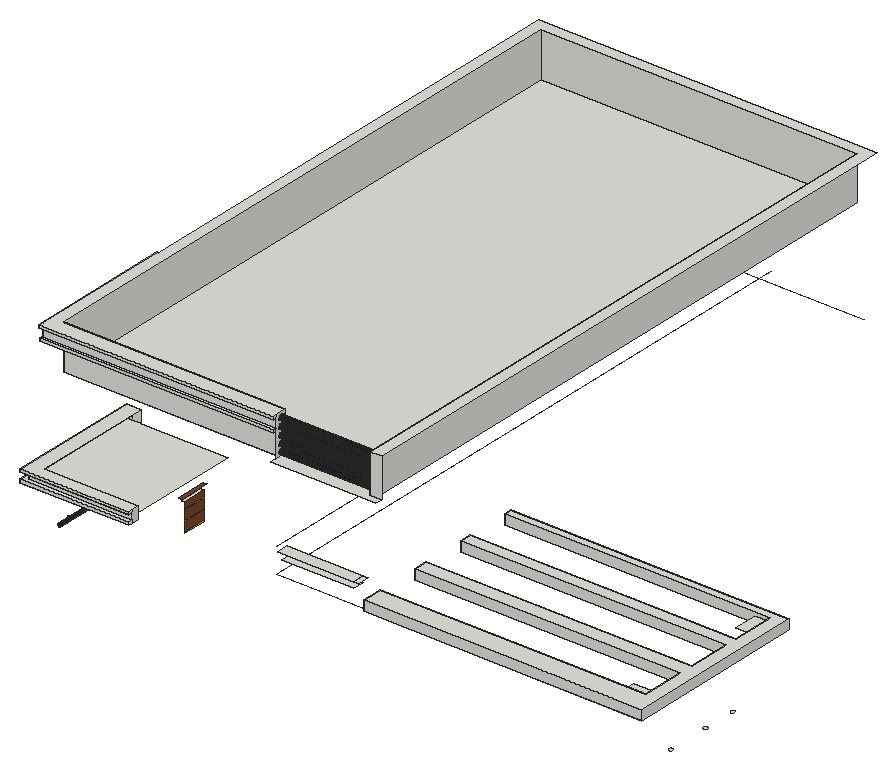
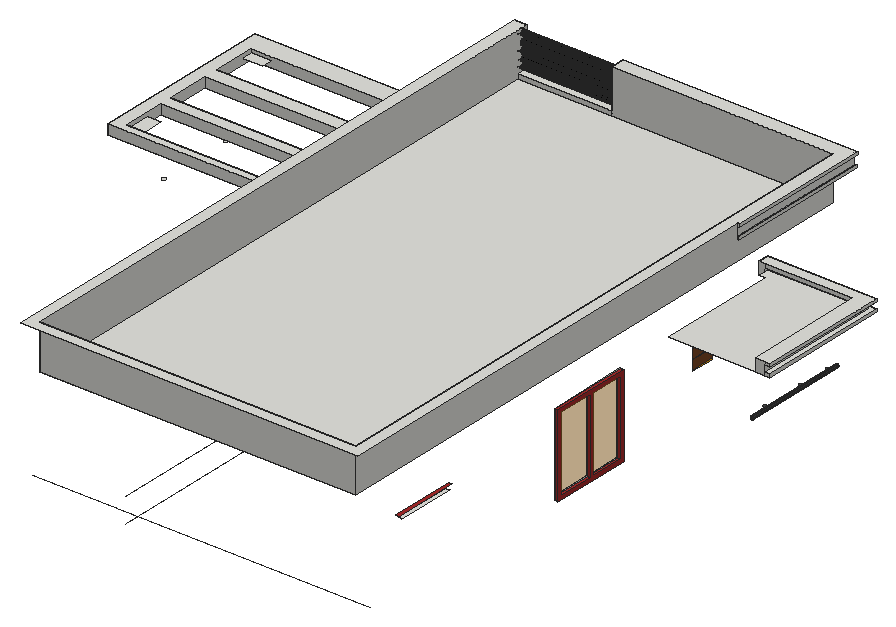
# SketchUp Ruby script. Lengths in inches.
U = 1.inch
M = Sketchup.active_model
def pt(a) = Geom::Point3d.new(a.map { |v| v * U })
def face(e, loops, mat)
  f = e.add_face(loops[0].map { |a| pt(a) })
  loops[1..].each { |l| e.add_face(l.map { |a| pt(a) }).erase! }
  f.material = f.back_material = mat if mat
  f
end
# faces: each face lists its corners as indices into pts; further lists are holes
def faces(e, pts, list, mat = nil) = list.each { |f| face(e, (f[0].is_a?(Array) ? f : [f]).map { |l| l.map { |i| pts[i] } }, mat) }
# xy, xz, yz: faces in a plane at the given z, y or x. An outline is a flat list of corners, or four numbers for a rectangle; further outlines are holes
def ring(l) = l.size == 4 ? [[l[0], l[1]], [l[2], l[1]], [l[2], l[3]], [l[0], l[3]]] : l.each_slice(2).to_a
def flat(e, list, mat, &to3) = list.each { |f| face(e, (f[0].is_a?(Array) ? f : [f]).map { |l| ring(l).map { |u, v| to3.(u, v) } }, mat) }
def xy(e, z, list, mat = nil) = flat(e, list, mat) { |x, y| [x, y, z] }
def xz(e, y, list, mat = nil) = flat(e, list, mat) { |x, z| [x, y, z] }
def yz(e, x, list, mat = nil) = flat(e, list, mat) { |y, z| [x, y, z] }
def lines(e, pts, list) = list.each { |a, b| e.add_line(pt(pts[a]), pt(pts[b])) }
# prism: a flat outline (further loops are holes) pulled along v
def prism(e, loops, v, mat = nil)
  f = face(e, loops, mat); d = Geom::Vector3d.new(v.map { |x| x * U })
  f.pushpull(f.normal.samedirection?(d) ? d.length : -d.length)
end
def box(e, o, s, mat = nil) = prism(e, [[o, [o[0] + s[0], o[1], o[2]], [o[0] + s[0], o[1] + s[1], o[2]], [o[0], o[1] + s[1], o[2]]]], [0, 0, s[2]], mat)
def at(x, y, z, deg = 0) = Geom::Transformation.translation(pt([x, y, z])) * Geom::Transformation.rotation(ORIGIN, Z_AXIS, deg.degrees)
def axes(o, x, y, z) = Geom::Transformation.new([*x, 0, *y, 0, *z, 0, *pt(o).to_a, 1])
def part(name) = M.definitions.add(name)
# library, detail: a bought-in or finely detailed component or shape, given as its bounding box
def library(name, o, s) = part(name).tap { |d| box(d.entities, o, s) }
def detail(e, o, s) = box(e.add_group.entities, o, s)
def put(e, d, t, mat = nil) = e.add_instance(d, t).tap { |i| i.material = mat if mat }
def group(e, t, mat = nil) = e.add_group.tap { |g| g.transformation = t; g.material = mat if mat }.entities
root = M.entities
M.materials.add("[0018_Brown]").color = [165, 42, 42]
M.materials.add("[0038_Orange]").color = [255, 165, 0]
M.materials.add("[0137_Black]").color = [71, 71, 71]
M.materials.add("[0137_Black]1").color = [0, 0, 0]
M.materials.add("[Translucent Glass Gray]").color = [191, 123, 24]
M.materials["[Translucent Glass Gray]"].alpha = 0.5
M.materials.add("[Wood Veneer 01]").color = [120, 70, 37]
prism(root,[[[512.421,0,493.967],[286.171,0,493.967],[286.171,12.1875,493.967],[286.171,16.939,493.967],[501.796,16.939,493.967],[501.796,51.752,493.967],[286.171,51.752,493.967],[286.171,63.752,493.967],[501.796,63.752,493.967],[501.796,98.564,493.967],[286.171,98.564,493.967],[286.171,108.439,493.967],[501.796,108.439,493.967],[501.796,143.252,493.967],[286.171,143.252,493.967],[286.171,149.476,493.967],[512.421,149.476,493.967]]],[0,0,8])
xy(root,448.181,[[499.408,44.29,499.78,44.339,500.127,44.482,500.424,44.711,500.653,45.008,500.796,45.355,500.845,45.727,500.796,46.099,500.653,46.446,500.424,46.744,500.127,46.972,499.78,47.116,499.408,47.165,499.036,47.116,498.689,46.972,498.391,46.744,498.163,46.446,498.019,46.099,497.97,45.727,498.019,45.355,498.163,45.008,498.391,44.711,498.689,44.482,499.036,44.339],[499.408,79.415,499.78,79.464,500.127,79.607,500.424,79.836,500.653,80.133,500.796,80.48,500.845,80.852,500.796,81.224,500.653,81.571,500.424,81.869,500.127,82.097,499.78,82.241,499.408,82.29,499.036,82.241,498.689,82.097,498.391,81.869,498.163,81.571,498.019,81.224,497.97,80.852,498.019,80.48,498.163,80.133,498.391,79.836,498.689,79.607,499.036,79.464],[499.408,107.04,499.78,107.089,500.127,107.232,500.424,107.461,500.653,107.758,500.796,108.105,500.845,108.477,500.796,108.849,500.653,109.196,500.424,109.494,500.127,109.722,499.78,109.866,499.408,109.915,499.036,109.866,498.689,109.722,498.391,109.494,498.163,109.196,498.019,108.849,497.97,108.477,498.019,108.105,498.163,107.758,498.391,107.461,498.689,107.232,499.036,107.089]])
xy(root,450.401,[[15.224,38.964,15.465,38.996,15.69,39.089,15.882,39.237,16.03,39.429,16.123,39.654,16.155,39.895,16.123,40.135,16.03,40.36,15.882,40.552,15.69,40.7,15.465,40.793,15.224,40.825,14.984,40.793,14.759,40.7,14.566,40.552,14.419,40.36,14.326,40.135,14.294,39.895,14.326,39.654,14.419,39.429,14.566,39.237,14.759,39.089,14.984,38.996],[15.849,65.839,16.09,65.871,16.315,65.964,16.507,66.112,16.655,66.304,16.748,66.529,16.78,66.77,16.748,67.01,16.655,67.235,16.507,67.427,16.315,67.575,16.09,67.668,15.849,67.7,15.609,67.668,15.384,67.575,15.191,67.427,15.044,67.235,14.951,67.01,14.919,66.77,14.951,66.529,15.044,66.304,15.191,66.112,15.384,65.964,15.609,65.871],[15.849,101.902,16.09,101.933,16.315,102.026,16.507,102.174,16.655,102.367,16.748,102.591,16.78,102.832,16.748,103.073,16.655,103.297,16.507,103.49,16.315,103.638,16.09,103.731,15.849,103.762,15.609,103.731,15.384,103.638,15.191,103.49,15.044,103.297,14.951,103.073,14.919,102.832,14.951,102.591,15.044,102.367,15.191,102.174,15.384,102.026,15.609,101.933]],"[0137_Black]")
xy(root,470.089,[[79.845,73.086,82.845,92.211]])
xy(root,473.089,[[79.845,70.086,82.845,95.211]],"[Wood Veneer 01]")
xy(root,479.029,[[8.875,254.471,11.875,321.346]],"[0018_Brown]")
xy(root,482.029,[[8.875,257.471,11.875,285.627],[8.875,287.909,11.875,318.346]],"[0018_Brown]")
xy(root,483,[[[0,9.1875,0,117.1875,11.875,117.1875,11.875,116.75,82.845,116.75,82.845,18.1875,88.408,18.1875,88.408,9.1875],[11.9375,19,16.875,30.25]],[11.9375,19,16.875,30.25],[284.046,22.046,284.046,22.066,284.415,22.0625,285.29,22.0625,285.29,22.054,286.171,22.046],[284.046,22.046,284.415,22.054],[284.415,22.046,285.29,22.054],
  [285.29,22.046,286.171,22.046,285.29,22.054],[284.046,22.054,284.415,22.0625],[284.415,22.054,285.29,22.054,284.415,22.0625],[285.29,22.054,285.29,22.0625,284.415,22.0625],[284.046,22.0625,284.415,22.0625,284.046,22.066]])
xy(root,485.689,[[0,9.1875,88.408,9.1875,88.408,12.1875,4.125,12.1875,4.125,117.1875,0,117.1875]])
xy(root,490.904,[[0,9.1875,0,117.1875,4.125,117.1875,4.125,12.1875,88.408,12.1875,88.408,9.1875]])
xy(root,493.0625,[[0,9.1875,88.408,9.1875,88.408,18.1875,11.875,18.1875,11.875,117.1875,0,117.1875]])
xy(root,499.431,[[484.5625,1.0625,510.6875,26.4375],[490.125,122.75,510.6875,143.77]])
xy(root,505.684,[[217.107,3.1875,275.758,12.1875]])
xy(root,510.503,[[213.982,3.1875,275.758,12.1875]])
xy(root,510.53,[[275.758,3.1875,279.919,12.1875]])
xy(root,536.147,[[8.875,431.778,11.875,479.716]])
xy(root,539.147,[[8.875,428.778,11.875,482.716]],"[0018_Brown]")
xy(root,542.904,[[8.875,257.471,11.875,285.627],[8.875,287.909,11.875,318.346]],"[0018_Brown]")
xy(root,545.904,[[8.875,254.471,11.875,321.346]],"[0018_Brown]")
xy(root,563.125,[[20.875,27.1875,277.171,511.875]])
xy(root,567.219,[[200.791,12.1875,286.171,12.1875,286.171,18.1875,277.171,18.1875,277.171,27.1875,200.791,27.1875]])
xy(root,587.3125,[[10.75,15.1875,10.75,135.0625,11.875,135.0625,11.875,18.1875,200.791,18.1875,200.791,15.1875]])
xy(root,589.538,[[10.75,15.1875,200.791,15.1875,200.791,17.5625,11.875,17.5625,11.875,135.0625,10.75,135.0625],[11.875,17.5625,200.791,18.1875]])
xy(root,596.571,[[10.25,15.1875,10.25,135.0625,11.875,135.0625,11.875,17.5625,200.791,17.5625,200.791,15.1875]])
xy(root,599.125,[[10.25,15.1875,200.791,15.1875,200.791,27.1875,20.875,27.1875,20.875,511.875,277.171,511.875,277.171,18.1875,286.171,18.1875,286.171,520.875,11.875,520.875,11.875,135.0625,10.25,135.0625]])
xz(root,9.1875,[[0,483,88.408,485.689],[0,490.904,88.408,493.0625]])
xz(root,12.1875,[[4.125,485.689,88.408,490.904]])
xz(root,15.1875,[[10.75,587.3125,200.791,589.538],[10.25,596.571,200.791,599.125]])
xz(root,17.5625,[[11.875,589.538,200.791,596.571]])
xz(root,18.1875,[[277.171,567.219,286.171,599.125],[11.875,587.243,200.791,587.3125],[11.875,587.3125,200.791,589.538]])
xz(root,27.1875,[[20.875,563.125,200.791,599.125],[200.791,563.125,277.171,567.219]])
xz(root,117.1875,[[0,483,4.125,485.689],[4.125,483,11.875,493.0625],[0,490.904,4.125,493.0625]])
xz(root,135.0625,[[10.75,587.3125,11.875,589.538],[10.25,596.571,11.875,599.125]])
xz(root,254.471,[[8.875,479.029,11.875,545.904]],"[0018_Brown]")
xz(root,257.471,[[8.875,482.029,11.875,542.904]],"[0018_Brown]")
xz(root,285.627,[[8.875,482.029,11.875,542.904]],"[0018_Brown]")
xz(root,287.909,[[8.875,482.029,11.875,542.904]],"[0018_Brown]")
xz(root,318.346,[[8.875,482.029,11.875,542.904]],"[0018_Brown]")
xz(root,321.346,[[8.875,479.029,11.875,545.904]],"[0018_Brown]")
xz(root,511.875,[[20.875,563.125,277.171,599.125]])
yz(root,0,[[9.1875,483,117.1875,485.689],[9.1875,490.904,117.1875,493.0625]])
yz(root,4.125,[[12.1875,485.689,117.1875,490.904]])
yz(root,8.875,[[[254.471,479.029,321.346,545.904],[287.909,482.029,318.346,542.904],[257.471,482.029,285.627,542.904]]],"[0018_Brown]")
yz(root,10.25,[[15.1875,596.571,135.0625,599.125]])
yz(root,10.75,[[15.1875,587.3125,135.0625,589.538]])
yz(root,11.875,[[[254.471,479.029,321.346,545.904],[287.909,482.029,318.346,542.904],[257.471,482.029,285.627,542.904]],[18.1875,587.3125,135.0625,589.538],[17.5625,589.538,135.0625,596.571]])
yz(root,11.875,[[257.471,482.029,285.627,542.904],[287.909,482.029,318.346,542.904]],"[Translucent Glass Gray]")
yz(root,20.875,[[27.1875,563.125,511.875,599.125]])
yz(root,82.845,[[73.086,447.376,92.211,448.489],[73.086,455.688,92.211,456.802],[73.086,464.001,92.211,465.114]],"[0038_Orange]")
yz(root,82.845,[[73.086,448.489,92.211,455.688],[73.086,456.802,92.211,464.001],[73.086,465.114,92.211,470.089]],"[Wood Veneer 01]")
yz(root,88.408,[[9.1875,483,12.1875,485.689],[12.1875,483,18.1875,493.0625],[9.1875,490.904,12.1875,493.0625]])
yz(root,200.791,[[[18.1875,567.219,27.1875,567.219,27.1875,599.125,18.1875,599.125,18.1875,596.571,17.5625,596.571,17.5625,589.538,18.1875,589.538],[22.313,593.302,21.763,593.374,21.251,593.586,20.811,593.924,20.473,594.364,20.261,594.877,20.188,595.427,20.261,595.977,20.473,596.489,20.811,596.929,21.251,597.267,21.763,597.479,22.313,597.552,22.863,597.479,23.376,597.267,23.816,596.929,24.154,596.489,24.366,595.977,24.438,595.427,24.366,594.877,24.154,594.364,23.816,593.924,23.376,593.586,22.863,593.374],[22.313,587.052,21.763,587.124,21.251,587.336,20.811,587.674,20.473,588.114,20.261,588.627,20.188,589.177,20.261,589.727,20.473,590.239,20.811,590.679,21.251,591.017,21.763,591.229,22.313,591.302,22.863,591.229,23.376,591.017,23.816,590.679,24.154,590.239,24.366,589.727,24.438,589.177,24.366,588.627,24.154,588.114,23.816,587.674,23.376,587.336,22.863,587.124],[22.313,580.802,21.763,580.874,21.251,581.086,20.811,581.424,20.473,581.864,20.261,582.377,20.188,582.927,20.261,583.477,20.473,583.989,20.811,584.429,21.251,584.767,21.763,584.979,22.313,585.052,22.863,584.979,23.376,584.767,23.816,584.429,24.154,583.989,24.366,583.477,24.438,582.927,24.366,582.377,24.154,581.864,23.816,581.424,23.376,581.086,22.863,580.874],[22.313,574.552,21.763,574.624,21.251,574.836,20.811,575.174,20.473,575.614,20.261,576.127,20.188,576.677,20.261,577.227,20.473,577.739,20.811,578.179,21.251,578.517,21.763,578.729,22.313,578.802,22.863,578.729,23.376,578.517,23.816,578.179,24.154,577.739,24.366,577.227,24.438,576.677,24.366,576.127,24.154,575.614,23.816,575.174,23.376,574.836,22.863,574.624]],[15.1875,587.3125,18.1875,589.538],[15.1875,596.571,18.1875,599.125]])
yz(root,275.758,[[3.1875,510.503,12.1875,510.53]])
yz(root,277.171,[[[27.1875,563.125,27.1875,567.219,18.1875,567.219,18.1875,599.125,511.875,599.125,511.875,563.125],[22.313,587.052,22.863,587.124,23.376,587.336,23.816,587.674,24.154,588.114,24.366,588.627,24.438,589.177,24.366,589.727,24.154,590.239,23.816,590.679,23.376,591.017,22.863,591.229,22.313,591.302,21.763,591.229,21.251,591.017,20.811,590.679,20.473,590.239,20.261,589.727,20.188,589.177,20.261,588.627,20.473,588.114,20.811,587.674,21.251,587.336,21.763,587.124]]])
yz(root,279.354,[[22.313,574.552,22.863,574.624,23.376,574.836,23.816,575.174,24.154,575.614,24.366,576.127,24.438,576.677,24.366,577.227,24.154,577.739,23.816,578.179,23.376,578.517,22.863,578.729,22.313,578.802,21.763,578.729,21.251,578.517,20.811,578.179,20.473,577.739,20.261,577.227,20.188,576.677,20.261,576.127,20.473,575.614,20.811,575.174,21.251,574.836,21.763,574.624],[22.313,580.802,22.863,580.874,23.376,581.086,23.816,581.424,24.154,581.864,24.366,582.377,24.438,582.927,24.366,583.477,24.154,583.989,23.816,584.429,23.376,584.767,22.863,584.979,22.313,585.052,21.763,584.979,21.251,584.767,20.811,584.429,20.473,583.989,20.261,583.477,20.188,582.927,20.261,582.377,20.473,581.864,20.811,581.424,21.251,581.086,21.763,580.874]])
yz(root,279.416,[[22.313,593.302,22.863,593.374,23.376,593.586,23.816,593.924,24.154,594.364,24.366,594.877,24.438,595.427,24.366,595.977,24.154,596.489,23.816,596.929,23.376,597.267,22.863,597.479,22.313,597.552,21.763,597.479,21.251,597.267,20.811,596.929,20.473,596.489,20.261,595.977,20.188,595.427,20.261,594.877,20.473,594.364,20.811,593.924,21.251,593.586,21.763,593.374]])
p = [[14.598,30.25,447.006],[14.311,30.25,447.125],[14.311,116.75,447.125],[14.598,116.75,447.006],[14.905,30.25,446.966],[14.905,116.75,446.966],
  [15.212,30.25,447.006],[15.212,116.75,447.006],[15.499,30.25,447.125],[15.499,116.75,447.125],[14.065,30.25,447.314],[14.065,116.75,447.314],
  [15.745,30.25,447.314],[15.745,116.75,447.314],[13.876,30.25,447.56],[13.876,116.75,447.56],[15.933,30.25,447.56],[15.933,116.75,447.56],
  [13.758,30.25,447.846],[13.758,116.75,447.846],[16.052,30.25,447.846],[16.052,116.75,447.846],[13.717,30.25,448.153],[13.717,116.75,448.153],
  [16.092,30.25,448.153],[16.092,116.75,448.153],[13.758,30.25,448.461],[13.758,116.75,448.461],[16.052,30.25,448.461],[16.052,116.75,448.461],
  [13.876,30.25,448.747],[13.876,116.75,448.747],[15.933,30.25,448.747],[15.933,116.75,448.747],[14.065,30.25,448.993],[14.065,116.75,448.993],
  [15.745,30.25,448.993],[15.745,116.75,448.993],[14.311,30.25,449.182],[14.311,116.75,449.182],[15.499,30.25,449.182],[15.499,116.75,449.182],
  [14.598,30.25,449.3],[14.598,116.75,449.3],[15.212,30.25,449.3],[15.212,116.75,449.3],[14.905,30.25,449.341],[14.905,116.75,449.341],
  [200.791,21.763,569.062],[200.791,22.313,568.989],[279.354,22.313,568.989],[279.354,21.763,569.062],[200.791,22.863,569.062],[279.354,22.863,569.062],
  [200.791,21.251,569.274],[279.354,21.251,569.274],[200.791,23.376,569.274],[279.354,23.376,569.274],[200.791,20.811,569.612],[279.354,20.811,569.612],
  [200.791,23.816,569.612],[279.354,23.816,569.612],[200.791,20.473,570.052],[279.354,20.473,570.052],[200.791,24.154,570.052],[279.354,24.154,570.052],
  [200.791,20.261,570.564],[279.354,20.261,570.564],[200.791,24.366,570.564],[279.354,24.366,570.564],[200.791,20.188,571.114],[279.354,20.188,571.114],
  [200.791,24.438,571.114],[279.354,24.438,571.114],[200.791,20.261,571.664],[279.354,20.261,571.664],[200.791,24.366,571.664],[279.354,24.366,571.664],
  [200.791,20.473,572.177],[279.354,20.473,572.177],[200.791,24.154,572.177],[279.354,24.154,572.177],[200.791,20.811,572.617],[279.354,20.811,572.617],
  [200.791,23.816,572.617],[279.354,23.816,572.617],[200.791,21.251,572.954],[279.354,21.251,572.954],[200.791,23.376,572.954],[279.354,23.376,572.954],
  [200.791,21.763,573.167],[279.354,21.763,573.167],[200.791,22.863,573.167],[279.354,22.863,573.167],[200.791,22.313,573.239],[279.354,22.313,573.239],
  [200.791,21.251,574.836],[200.791,21.763,574.624],[279.354,21.763,574.624],[279.354,21.251,574.836],[200.791,22.313,574.552],[279.354,22.313,574.552],
  [200.791,22.863,574.624],[279.354,22.863,574.624],[200.791,23.376,574.836],[279.354,23.376,574.836],[200.791,20.811,575.174],[279.354,20.811,575.174],
  [200.791,23.816,575.174],[279.354,23.816,575.174],[200.791,20.473,575.614],[279.354,20.473,575.614],[200.791,24.154,575.614],[279.354,24.154,575.614],
  [200.791,20.261,576.127],[279.354,20.261,576.127],[200.791,24.366,576.127],[279.354,24.366,576.127],[200.791,20.188,576.677],[279.354,20.188,576.677],
  [200.791,24.438,576.677],[279.354,24.438,576.677],[200.791,20.261,577.227],[279.354,20.261,577.227],[200.791,24.366,577.227],[279.354,24.366,577.227],
  [200.791,20.473,577.739],[279.354,20.473,577.739],[200.791,24.154,577.739],[279.354,24.154,577.739],[200.791,20.811,578.179],[279.354,20.811,578.179],
  [200.791,23.816,578.179],[279.354,23.816,578.179],[200.791,21.251,578.517],[279.354,21.251,578.517],[200.791,23.376,578.517],[279.354,23.376,578.517],
  [200.791,21.763,578.729],[279.354,21.763,578.729],[200.791,22.863,578.729],[279.354,22.863,578.729],[200.791,22.313,578.802],[279.354,22.313,578.802],
  [200.791,21.763,580.874],[200.791,22.313,580.802],[279.354,22.313,580.802],[279.354,21.763,580.874],[200.791,22.863,580.874],[279.354,22.863,580.874],
  [200.791,21.251,581.086],[279.354,21.251,581.086],[200.791,23.376,581.086],[279.354,23.376,581.086],[200.791,20.811,581.424],[279.354,20.811,581.424],
  [200.791,23.816,581.424],[279.354,23.816,581.424],[200.791,20.473,581.864],[279.354,20.473,581.864],[200.791,24.154,581.864],[279.354,24.154,581.864],
  [200.791,20.261,582.377],[279.354,20.261,582.377],[200.791,24.366,582.377],[279.354,24.366,582.377],[200.791,20.188,582.927],[279.354,20.188,582.927],
  [200.791,24.438,582.927],[279.354,24.438,582.927],[200.791,20.261,583.477],[279.354,20.261,583.477],[200.791,24.366,583.477],[279.354,24.366,583.477],
  [200.791,20.473,583.989],[279.354,20.473,583.989],[200.791,24.154,583.989],[279.354,24.154,583.989],[200.791,20.811,584.429],[279.354,20.811,584.429],
  [200.791,23.816,584.429],[279.354,23.816,584.429],[200.791,21.251,584.767],[279.354,21.251,584.767],[200.791,23.376,584.767],[279.354,23.376,584.767],
  [200.791,21.763,584.979],[279.354,21.763,584.979],[200.791,22.863,584.979],[279.354,22.863,584.979],[200.791,22.313,585.052],[279.354,22.313,585.052],
  [200.791,21.251,587.336],[200.791,21.763,587.124],[277.171,21.763,587.124],[277.171,21.251,587.336],[200.791,22.313,587.052],[277.171,22.313,587.052],
  [200.791,22.863,587.124],[277.171,22.863,587.124],[200.791,23.376,587.336],[277.171,23.376,587.336],[200.791,20.811,587.674],[277.171,20.811,587.674],
  [200.791,23.816,587.674],[277.171,23.816,587.674],[200.791,20.473,588.114],[277.171,20.473,588.114],[200.791,24.154,588.114],[277.171,24.154,588.114],
  [200.791,20.261,588.627],[277.171,20.261,588.627],[200.791,24.366,588.627],[277.171,24.366,588.627],[200.791,20.188,589.177],[277.171,20.188,589.177],
  [200.791,24.438,589.177],[277.171,24.438,589.177],[200.791,20.261,589.727],[277.171,20.261,589.727],[200.791,24.366,589.727],[277.171,24.366,589.727],
  [200.791,20.473,590.239],[277.171,20.473,590.239],[200.791,24.154,590.239],[277.171,24.154,590.239],[200.791,20.811,590.679],[277.171,20.811,590.679],
  [200.791,23.816,590.679],[277.171,23.816,590.679],[200.791,21.251,591.017],[277.171,21.251,591.017],[200.791,23.376,591.017],[277.171,23.376,591.017],
  [200.791,21.763,591.229],[277.171,21.763,591.229],[200.791,22.863,591.229],[277.171,22.863,591.229],[200.791,22.313,591.302],[277.171,22.313,591.302],
  [200.791,21.763,593.374],[200.791,22.313,593.302],[279.416,22.313,593.302],[279.416,21.763,593.374],[200.791,22.863,593.374],[279.416,22.863,593.374],
  [200.791,21.251,593.586],[279.416,21.251,593.586],[200.791,23.376,593.586],[279.416,23.376,593.586],[200.791,20.811,593.924],[279.416,20.811,593.924],
  [200.791,23.816,593.924],[279.416,23.816,593.924],[200.791,20.473,594.364],[279.416,20.473,594.364],[200.791,24.154,594.364],[279.416,24.154,594.364],
  [200.791,20.261,594.877],[279.416,20.261,594.877],[200.791,24.366,594.877],[279.416,24.366,594.877],[200.791,20.188,595.427],[279.416,20.188,595.427],
  [200.791,24.438,595.427],[279.416,24.438,595.427],[200.791,20.261,595.977],[279.416,20.261,595.977],[200.791,24.366,595.977],[279.416,24.366,595.977],
  [200.791,20.473,596.489],[279.416,20.473,596.489],[200.791,24.154,596.489],[279.416,24.154,596.489],[200.791,20.811,596.929],[279.416,20.811,596.929],
  [200.791,23.816,596.929],[279.416,23.816,596.929],[200.791,21.251,597.267],[279.416,21.251,597.267],[200.791,23.376,597.267],[279.416,23.376,597.267],
  [200.791,21.763,597.479],[279.416,21.763,597.479],[200.791,22.863,597.479],[279.416,22.863,597.479],[200.791,22.313,597.552],[279.416,22.313,597.552],
  [200.791,18.1875,483],[286.171,18.1875,483],[200.791,508.3125,483],[200.791,18.1875,503.125],[200.791,520.875,503.125],[11.875,30.25,483],
  [11.9375,30.25,483],[4.125,12.1875,483],[4.125,12.1875,485.689],[275.758,12.1875,505.684],[275.758,12.1875,510.503],[11.875,508.3125,483],
  [286.171,508.3125,483],[200.791,520.875,483],[11.875,18.1875,596.571],[11.875,18.1875,599.125]]
faces(root,p,[[0,1,2,3],[4,0,3,5],[6,4,5,7],[8,6,7,9],[1,10,11,2],[12,8,9,13],[10,14,15,11],[16,12,13,17],
  [14,18,19,15],[20,16,17,21],[18,22,23,19],[24,20,21,25],[22,26,27,23],[28,24,25,29],[26,30,31,27],[32,28,29,33],
  [30,34,35,31],[36,32,33,37],[34,38,39,35],[40,36,37,41],[38,42,43,39],[44,40,41,45],[42,46,47,43],[46,44,45,47]],"[0137_Black]")
faces(root,p,[[48,49,50,51],[49,52,53,50],[54,48,51,55],[52,56,57,53],[58,54,55,59],[56,60,61,57],[62,58,59,63],[60,64,65,61],
  [66,62,63,67],[64,68,69,65],[70,66,67,71],[68,72,73,69],[74,70,71,75],[72,76,77,73],[78,74,75,79],[76,80,81,77],
  [82,78,79,83],[80,84,85,81],[86,82,83,87],[84,88,89,85],[90,86,87,91],[88,92,93,89],[94,90,91,95],[92,94,95,93],
  [96,97,98,99],[97,100,101,98],[100,102,103,101],[102,104,105,103],[106,96,99,107],[104,108,109,105],[110,106,107,111],[108,112,113,109],
  [114,110,111,115],[112,116,117,113],[118,114,115,119],[116,120,121,117],[122,118,119,123],[120,124,125,121],[126,122,123,127],[124,128,129,125],
  [130,126,127,131],[128,132,133,129],[134,130,131,135],[132,136,137,133],[138,134,135,139],[136,140,141,137],[142,138,139,143],[140,142,143,141],
  [144,145,146,147],[145,148,149,146],[150,144,147,151],[148,152,153,149],[154,150,151,155],[152,156,157,153],[158,154,155,159],[156,160,161,157],
  [162,158,159,163],[160,164,165,161],[166,162,163,167],[164,168,169,165],[170,166,167,171],[168,172,173,169],[174,170,171,175],[172,176,177,173],
  [178,174,175,179],[176,180,181,177],[182,178,179,183],[180,184,185,181],[186,182,183,187],[184,188,189,185],[190,186,187,191],[188,190,191,189],
  [192,193,194,195],[193,196,197,194],[196,198,199,197],[198,200,201,199],[202,192,195,203],[200,204,205,201],[206,202,203,207],[204,208,209,205],
  [210,206,207,211],[208,212,213,209],[214,210,211,215],[212,216,217,213],[218,214,215,219],[216,220,221,217],[222,218,219,223],[220,224,225,221],
  [226,222,223,227],[224,228,229,225],[230,226,227,231],[228,232,233,229],[234,230,231,235],[232,236,237,233],[238,234,235,239],[236,238,239,237],
  [240,241,242,243],[241,244,245,242],[246,240,243,247],[244,248,249,245],[250,246,247,251],[248,252,253,249],[254,250,251,255],[252,256,257,253],
  [258,254,255,259],[256,260,261,257],[262,258,259,263],[260,264,265,261],[266,262,263,267],[264,268,269,265],[270,266,267,271],[268,272,273,269],
  [274,270,271,275],[272,276,277,273],[278,274,275,279],[276,280,281,277],[282,278,279,283],[280,284,285,281],[286,282,283,287],[284,286,287,285]],"[0137_Black]1")
lines(root,p,[[288,289],[288,290],[291,292],[293,294],[295,296],[297,298],[299,290],[290,300],[290,301],[302,303]])
